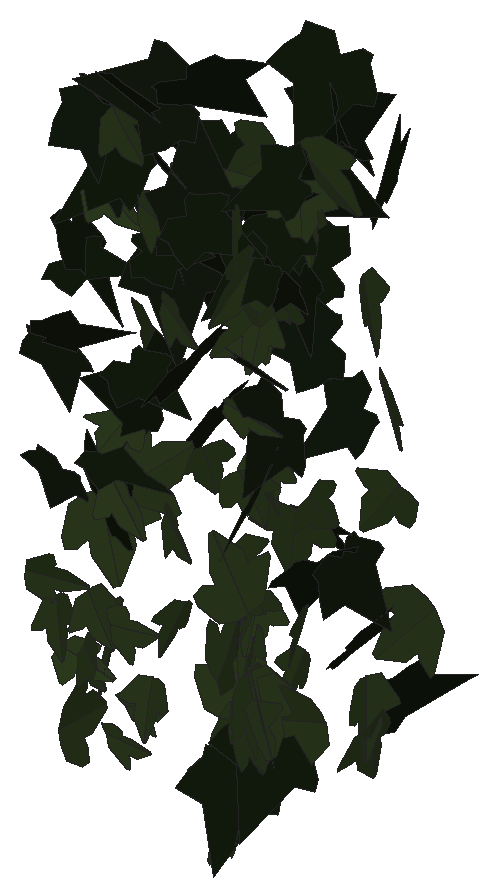
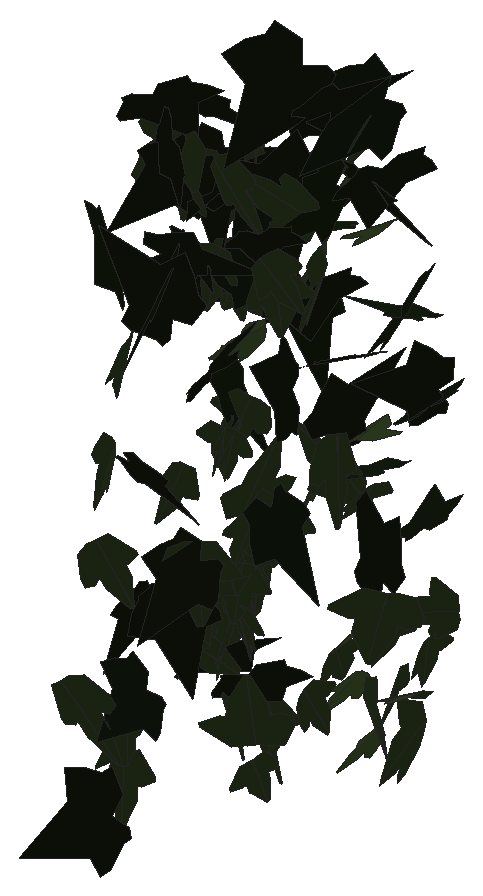
# SketchUp Ruby script. Lengths in inches.
U = 1.inch
M = Sketchup.active_model
def pt(a) = Geom::Point3d.new(a.map { |v| v * U })
def face(e, loops, mat)
  f = e.add_face(loops[0].map { |a| pt(a) })
  loops[1..].each { |l| e.add_face(l.map { |a| pt(a) }).erase! }
  f.material = f.back_material = mat if mat
  f
end
# faces: each face lists its corners as indices into pts; further lists are holes
def faces(e, pts, list, mat = nil) = list.each { |f| face(e, (f[0].is_a?(Array) ? f : [f]).map { |l| l.map { |i| pts[i] } }, mat) }
# xy, xz, yz: faces in a plane at the given z, y or x. An outline is a flat list of corners, or four numbers for a rectangle; further outlines are holes
def ring(l) = l.size == 4 ? [[l[0], l[1]], [l[2], l[1]], [l[2], l[3]], [l[0], l[3]]] : l.each_slice(2).to_a
def flat(e, list, mat, &to3) = list.each { |f| face(e, (f[0].is_a?(Array) ? f : [f]).map { |l| ring(l).map { |u, v| to3.(u, v) } }, mat) }
def xy(e, z, list, mat = nil) = flat(e, list, mat) { |x, y| [x, y, z] }
def xz(e, y, list, mat = nil) = flat(e, list, mat) { |x, z| [x, y, z] }
def yz(e, x, list, mat = nil) = flat(e, list, mat) { |y, z| [x, y, z] }
def lines(e, pts, list) = list.each { |a, b| e.add_line(pt(pts[a]), pt(pts[b])) }
# prism: a flat outline (further loops are holes) pulled along v
def prism(e, loops, v, mat = nil)
  f = face(e, loops, mat); d = Geom::Vector3d.new(v.map { |x| x * U })
  f.pushpull(f.normal.samedirection?(d) ? d.length : -d.length)
end
def box(e, o, s, mat = nil) = prism(e, [[o, [o[0] + s[0], o[1], o[2]], [o[0] + s[0], o[1] + s[1], o[2]], [o[0], o[1] + s[1], o[2]]]], [0, 0, s[2]], mat)
def at(x, y, z, deg = 0) = Geom::Transformation.translation(pt([x, y, z])) * Geom::Transformation.rotation(ORIGIN, Z_AXIS, deg.degrees)
def axes(o, x, y, z) = Geom::Transformation.new([*x, 0, *y, 0, *z, 0, *pt(o).to_a, 1])
def part(name) = M.definitions.add(name)
# library, detail: a bought-in or finely detailed component or shape, given as its bounding box
def library(name, o, s) = part(name).tap { |d| box(d.entities, o, s) }
def detail(e, o, s) = box(e.add_group.entities, o, s)
def put(e, d, t, mat = nil) = e.add_instance(d, t).tap { |i| i.material = mat if mat }
def group(e, t, mat = nil) = e.add_group.tap { |g| g.transformation = t; g.material = mat if mat }.entities
root = M.entities
M.materials.add("efeu1").color = [18, 25, 13]
M.materials.add("efeu2").color = [43, 57, 29]
c1 = part("ivyleaf_10")
p = [[0,0.5,-0.03],[-0.0625,2.02,-0.43],[-0.19,2.01,-0.46],[-0.54,1.05,-0.29],[-0.52,0.625,-0.18],[-0.83,0.76,-0.28],
  [-1.16,0.64,-0.33],[-1.15,0.33,-0.24],[-0.77,-0.39,0.02],[-0.3,-0.51,0.16],[0.04,-0.48,0.23],[-0.02,2.01,-0.4375],
  [-0.06,2.01,-0.43],[0.04,-0.49,0.23],[0.67,-0.49,0.14],[1.38,0.36,-0.2],[1.375,0.51,-0.24],[0.81,0.65,-0.19],
  [0.62,0.59,-0.15],[0.6,1.09,-0.28],[0.5,1.23,-0.31]]
faces(c1.entities,p,[[0,1,2,3,4,5,6,7,8,9,10],[11,12,0,13,14,15,16,17,18,19,20]],"efeu2")
c2 = part("ivyleaf_9")
p = [[1.54,2.16,1.25],[1.36,2.04,1.19],[-0.21,0.99,0.68],[-0.71,1.11,0.82],[-0.85,0.86,0.67],[-0.8,0.17,0.21],
  [-0.9,-0.01,0.1],[-0.67,-0.16,-0.02],[-0.08,-0.08,-0.05],[-0.03,-0.6,-0.4],[0.65,-0.88,-0.66],[0.83,-0.6,-0.49],
  [1.29,-0.42,-0.43],[1.8125,-0.07,-0.26],[1.21,0.44,0.15]]
faces(c2.entities,p,[[0,1,2,3,4,5,6,7,8,9,10,11,12,13,14]],"efeu1")
put(root,c1,axes([586.05,128.29,189.875],[0.13777,-0.1156,0.68429],[0.55453,0.4378,-0.03769],[-0.41727,0.54365,0.17585]))
put(root,c1,axes([586.36,128.71,188.74],[-0.02608,-0.71977,0.14562],[0.34937,-0.14032,-0.63103],[0.64591,0.04684,0.3472]))
put(root,c2,axes([586.13,129.02,196.92],[0.02994,-0.77843,0.19838],[0.30223,-0.17302,-0.72452],[0.74429,0.10157,0.28622]))
put(root,c2,axes([586.26,129.04,192.97],[-0.21332,-0.59102,0.45433],[0.308,-0.50022,-0.5061],[0.67886,0.04124,0.37238]))
put(root,c2,axes([586.15,128.7,197.34],[0.47444,0.02155,0.66199],[0.63643,0.21069,-0.46298],[-0.18344,0.78673,0.10585]))
put(root,c1,axes([586.41,130.7,191.02],[0.78115,0.73417,0.24902],[0.18487,0.16692,-1.072],[-0.75289,0.80271,-0.00485]))
put(root,c1,axes([587.17,132.04,196.33],[-0.85539,0.2797,0.52223],[-0.49092,0.17874,-0.89983],[-0.3316,-0.98614,-0.01498]))
put(root,c2,axes([586.34,129.57,200.51],[0.65227,-0.79795,-0.17464],[-0.10982,0.1358,-1.03062],[0.80942,0.66145,0.00091]))
put(root,c1,axes([586.71,130.87,187.58],[0.69898,-0.74224,0.39536],[0.26843,-0.29029,-1.01955],[0.79698,0.74875,-0.00336]))
put(root,c1,axes([587.25,128.31,185.47],[-0.07423,0.16774,1.11083],[-0.49986,0.99205,-0.1832],[-1.00609,-0.50526,0.00907]))
put(root,c1,axes([586.64,129.05,187.25],[0.01692,-0.64732,-0.23753],[0.67208,0.06858,-0.13903],[0.1541,-0.22804,0.63244]))
put(root,c2,axes([586.54,129.05,199.8],[0.55427,-0.51643,-0.1309],[0.45505,0.55715,-0.27124],[0.27707,0.11807,0.70735]))
put(root,c1,axes([587.25,128.96,187.52],[0.25073,-0.64179,-0.17543],[0.26152,0.26745,-0.60466],[0.61178,0.1487,0.33037]))
put(root,c2,axes([586.82,130.28,191.63],[-0.13016,-0.00362,1.19027],[0.56176,-1.05581,0.05822],[1.04937,0.56476,0.11648]))
put(root,c2,axes([587.21,129.76,204.62],[-0.10832,-1.02535,-0.37043],[0.03645,0.36864,-1.03105],[1.0896,-0.11427,-0.00234]))
put(root,c1,axes([587.44,128.96,189.1875],[-0.05976,-0.73491,-0.09625],[0.43185,0.04395,-0.60374],[0.60238,-0.10442,0.42327]))
put(root,c1,axes([588.15,131.93,187.85],[-0.00093,-0.60937,0.30873],[0.04157,-0.30821,-0.60822],[0.68185,0.01797,0.0375]))
put(root,c2,axes([588.63,129.31,203.83],[-1.09293,0.11233,-0.02551],[0.01922,-0.06221,-1.09706],[-0.11357,-1.09146,0.0599]))
put(root,c1,axes([588.66,133.1,202.34],[0.48228,0.09622,-0.59732],[-0.59134,0.23653,-0.43934],[0.12797,0.73037,0.22098]))
put(root,c1,axes([587.73,129.0625,202.3],[0.02053,-0.78461,-0.03553],[0.75258,0.02982,-0.22368],[0.22472,-0.02819,0.75233]))
put(root,c1,axes([588.43,129.09,195.15],[-0.6903,-0.14918,0.224],[0.19282,-0.70434,0.12516],[0.18774,0.17491,0.69505]))
put(root,c2,axes([588.86,132.73,194.125],[-0.47604,0.80347,-0.50065],[0.23512,-0.44248,-0.93368],[-0.91702,-0.53054,0.0205]))
put(root,c1,axes([588.3,128.86,185.18],[0.52006,-0.39557,-0.21933],[0.30808,0.5545,-0.26956],[0.33116,0.10536,0.59521]))
put(root,c2,axes([587.97,128.91,194.15],[0.46394,-0.60081,-0.1519],[0.37966,0.42553,-0.52352],[0.48981,0.23925,0.54968]))
put(root,c2,axes([588.8125,130.11,195.7],[-0.01816,-0.01498,1.10733],[-0.71725,-0.84365,-0.02318],[0.84377,-0.71747,0.00413]))
put(root,c1,axes([588.78,132.73,201.58],[-0.57493,-0.49623,0.11289],[-0.03338,-0.13318,-0.75543],[0.50781,-0.57057,0.07815]))
put(root,c2,axes([587.9,133.13,198.65],[0.28392,-0.11605,-1.00857],[1.01522,0.03577,0.28167],[0.00321,-1.04716,0.12139]))
put(root,c2,axes([588.2,128.67,206.07],[1.12084,0.05707,0.01287],[0.01107,0.03564,-1.12175],[-0.05745,1.12035,0.03503]))
put(root,c1,axes([588.54,128.7,205.13],[0.09649,-0.7933,-0.18292],[0.45075,0.20545,-0.65323],[0.67795,-0.02369,0.46035]))
put(root,c1,axes([588.58,128.72,188.88],[0.46426,-0.3966,-0.40602],[0.32133,0.61605,-0.23433],[0.46785,-0.02956,0.56385]))
put(root,c1,axes([588.48,128.8,193.16],[-0.14155,-0.72801,-0.0542],[0.57266,-0.07649,-0.46817],[0.45276,-0.13085,0.5752]))
put(root,c1,axes([588.9,130.625,200.91],[-0.6167,0.84837,-0.22552],[0.15082,-0.16911,-1.0486],[-0.86478,-0.63449,-0.02206]))
put(root,c2,axes([589.65,130.02,205.68],[-0.12174,-0.90105,-0.60518],[-0.09557,-0.59771,0.90915],[-1.0812,0.15429,-0.01222]))
put(root,c1,axes([589.28,131.74,193.35],[-0.38397,-0.59309,-0.15346],[0.11431,0.10857,-0.70561],[0.60186,-0.399,0.03611]))
put(root,c1,axes([589.1875,128.57,186.6],[0.5933,-0.23635,-0.26569],[0.18712,0.64698,-0.1577],[0.30239,0.06339,0.61887]))
put(root,c2,axes([588.93,129.92,203.5625],[1.04486,-0.33971,-0.04287],[-0.04218,0.00891,-1.09869],[0.3398,1.04571,-0.00457]))
put(root,c2,axes([589.33,132.72,203.03],[-0.33806,-0.65558,-0.25431],[0.18801,0.18763,-0.73361],[0.67757,-0.37915,0.07668]))
put(root,c2,axes([589.27,130.45,200.19],[-0.17654,-1.02923,-0.21362],[0.03699,0.21039,-1.04426],[1.05052,-0.18037,0.00088]))
put(root,c2,axes([589.08,128.72,197.41],[0.32391,-0.6182,-0.31947],[0.34025,0.44809,-0.5221],[0.60701,0.07871,0.46313]))
put(root,c1,axes([588.9375,129.29,193.625],[0.67907,-0.13297,-0.79694],[0.79162,-0.09878,0.69102],[-0.16165,-1.04235,0.03618]))
put(root,c1,axes([589.71,128.68,187.3],[-0.20403,-0.588,0.33927],[0.32561,-0.39561,-0.48984],[0.59568,0.01485,0.38396]))
put(root,c1,axes([589.67,128.5625,202.63],[0.43747,-0.56137,-0.35728],[0.3332,0.55491,-0.46391],[0.57599,0.10536,0.53972]))
put(root,c2,axes([589.8,136.45,203.11],[0.75781,-0.50642,-0.66784],[-0.55853,0.36617,-0.91143],[0.62491,0.94139,-0.00475]))
put(root,c2,axes([589.73,128.52,201.375],[0.73576,-0.18714,-0.20691],[0.0998,0.72152,-0.2977],[0.26053,0.25211,0.69839]))
put(root,c2,axes([589.65,136.52,202.01],[-0.06323,-0.05609,1.12568],[0.9616,-0.59077,0.02457],[0.58789,0.96028,0.08087]))
put(root,c1,axes([590.36,131.73,185.89],[0.93344,0.55515,-0.12163],[0.08905,0.08812,1.08564],[0.5613,-0.9372,0.03003]))
put(root,c1,axes([589.8125,130.32,202.53],[0.3925,-0.06622,-1.01584],[1.01558,-0.04945,0.39562],[-0.07005,-1.0879,0.04385]))
put(root,c1,axes([590.48,128.57,192.98],[0.36868,-0.63247,-0.12508],[0.3146,0.30226,-0.60105],[0.56275,0.24539,0.41795]))
put(root,c2,axes([591.0625,129.26,202.32],[-1.14149,-0.10172,0.28438],[0.29042,-0.06455,1.14267],[-0.08289,1.17461,0.08742]))
put(root,c2,axes([590.49,129.54,206.7],[0.81903,0.87426,0.24465],[0.16851,0.17738,-1.19797],[-0.89207,0.83619,-0.00167]))
put(root,c1,axes([590.73,128.23,199.96],[0.4211,-0.63505,-0.13307],[0.38926,0.37418,-0.55389],[0.51911,0.23457,0.52328]))
put(root,c1,axes([591.51,131.55,203.77],[0.65074,-0.37421,-0.7487],[-0.66145,0.35123,-0.75045],[0.5129,0.92772,-0.01788]))
put(root,c2,axes([591.49,128.12,198.69],[-0.28552,1.10913,-0.1052],[0.02765,-0.10151,-1.14529],[-1.11377,-0.28685,-0.00146]))
put(root,c1,axes([591.19,130.65,183.99],[0.20398,0.59083,-0.20369],[-0.17534,-0.15155,-0.6152],[-0.59985,0.24521,0.11056]))
put(root,c1,axes([591.17,130.22,185.76],[0.54309,-0.39053,0.07419],[0.07251,-0.02619,-0.6686],[0.39085,0.54751,0.02094]))
put(root,c1,axes([591.41,129.73,185.25],[-0.37006,-0.55743,-0.02026],[0.01047,0.01737,-0.66908],[0.5577,-0.3702,-0.00088]))
put(root,c1,axes([591.66,132.8,191.61],[-0.89097,-0.38537,0.17041],[-0.132,-0.12326,-0.96889],[0.40016,-0.8987,0.05981]))
put(root,c1,axes([591.39,130.53,186.2],[0.62113,-0.25645,0.01845],[0.02071,0.00182,-0.67192],[0.25627,0.6214,0.00959]))
put(root,c1,axes([591.71,130.02,190.71],[-0.50006,0.4695,0.16327],[-0.16888,0.05736,-0.68216],[-0.46752,-0.5229,0.07177]))
put(root,c2,axes([591.41,133.0625,191.66],[0.9194,0.31654,-0.15049],[-0.1971,0.11759,-0.9568],[-0.28983,0.92418,0.17328]))
put(root,c1,axes([591.73,130.6875,190.12],[-0.63101,-0.29889,-0.0219],[0.01804,0.01306,-0.69821],[0.29915,-0.63126,-0.00408]))
put(root,c2,axes([590.97,130.36,200.35],[1.19253,-0.08387,-0.27225],[0.27139,-0.02173,1.19547],[-0.0866,-1.22302,-0.00257]))
put(root,c1,axes([591.83,130.93,185.69],[0.44027,-0.40444,-0.31148],[-0.20446,0.23719,-0.59697],[0.46775,0.48436,0.03224]))
put(root,c1,axes([591.64,130.63,188.6],[0.5263,-0.41905,0.14553],[0.12742,-0.07348,-0.67241],[0.42491,0.54108,0.02139]))
put(root,c1,axes([591.6875,130.67,188.92],[0.6654,-0.18185,0.0303],[0.0285,-0.01064,-0.6898],[0.18214,0.66601,-0.00275]))
put(root,c1,axes([591.74,130.23,191.66],[0.00038,0.65668,0.27499],[-0.06837,0.27376,-0.65363],[-0.70864,-0.02606,0.06321]))
put(root,c1,axes([591.8,130.83,189.76],[0.48171,0.48315,-0.13559],[-0.10284,-0.08891,-0.68219],[-0.49117,0.49247,0.00986]))
put(root,c2,axes([592.14,133.125,190.22],[0.12005,0.89185,-0.37066],[-0.11817,-0.35714,-0.8976],[-0.95855,0.15573,0.06423]))
put(root,c1,axes([592.24,129.09,191.43],[0.21223,-0.04077,-0.67789],[-0.4693,0.50456,-0.17727],[0.49088,0.5,0.12361]))
put(root,c1,axes([591.79,130.29,190.45],[0.6759,-0.17246,0.09423],[0.09296,-0.0168,-0.69752],[0.17315,0.68223,0.00664]))
put(root,c2,axes([591.35,128.43,203.07],[0.39277,-0.43328,-0.55246],[0.33174,0.67244,-0.29152],[0.61878,-0.08549,0.50696]))
put(root,c1,axes([591.97,129.75,189.73],[0.41568,-0.50478,-0.24792],[-0.0352,0.28433,-0.63794],[0.56127,0.39167,0.1436]))
put(root,c1,axes([591.55,129.53,185.12],[0.43241,-0.50984,-0.0235],[0.51036,0.43219,0.01431],[0.00428,-0.02717,0.66836]))
put(root,c1,axes([592.31,130.02,199.22],[0.51249,0.16623,-0.53106],[-0.5226,-0.10427,-0.53696],[-0.19118,0.73062,0.0442]))
put(root,c1,axes([591.81,130.79,185.48],[0.51009,-0.18841,0.39341],[0.38223,-0.09858,-0.54281],[0.21016,0.63659,0.03238]))
put(root,c1,axes([592.22,130.33,194.28],[-0.26185,0.67831,-0.02394],[0.00388,-0.02416,-0.72708],[-0.67872,-0.26183,0.00508]))
put(root,c1,axes([592.47,128.34,189.19],[0.01751,0.40215,-0.91438],[-0.09019,0.91142,0.39912],[0.99483,0.07555,0.05228]))
put(root,c2,axes([592.8,134.2,194.92],[-0.88282,0.07844,0.0797],[-0.07909,0.01043,-0.88629],[-0.07906,-0.88635,-0.00338]))
put(root,c1,axes([592.22,130.73,194.57],[0.71445,0.10714,0.07421],[0.06171,0.0861,-0.71847],[-0.1148,0.71312,0.0756]))
put(root,c1,axes([592.52,128.78,184.51],[0.80501,-0.64729,-0.2514],[-0.19611,0.1573,-1.03297],[0.66613,0.82856,-0.00029]))
put(root,c1,axes([592.5,129.94,200.125],[-0.73922,-0.1771,-0.04806],[0.04397,0.02274,-0.76005],[0.17816,-0.74044,-0.01185]))
put(root,c1,axes([592.44,130.39,194.54],[-0.32032,0.64019,0.12914],[-0.04323,0.12274,-0.71568],[-0.65165,-0.32283,-0.016]))
put(root,c2,axes([592.1875,136.14,184.4375],[0.42315,0.56634,0.87028],[0.5277,0.69207,-0.70694],[-0.89424,0.67638,-0.00536]))
put(root,c1,axes([592.47,130.07,199.4],[0.7576,0.01182,-0.00148],[-0.00148,0.00001,-0.75769],[-0.01182,0.7576,0.00003]))
put(root,c2,axes([592.65,133.92,187.4],[0.30197,0.62954,0.63039],[0.1013,0.63704,-0.6847],[-0.88513,0.28768,0.13671]))
put(root,c2,axes([593.4,131.97,200.66],[-0.7356,0.05233,0.71313],[-0.71484,-0.078,-0.73164],[0.0169,-1.02155,0.0924]))
put(root,c1,axes([592.78,130.49,200.06],[-0.75668,0.09692,0.02534],[-0.02567,-0.00091,-0.76285],[-0.09684,-0.7571,0.00416]))
put(root,c1,axes([592.82,128.76,191.35],[0.17805,1.02887,0.22739],[-0.04868,-0.22234,1.04411],[1.05257,-0.18432,0.00983]))
put(root,c1,axes([592.6,128.9,203.25],[-0.4011,0.46963,-0.48216],[0.14694,-0.48664,-0.59624],[-0.65684,-0.39565,0.16104]))
put(root,c2,axes([592.82,133.18,206.6],[-0.63802,-0.87666,-0.02225],[0.01293,0.01811,-1.08425],[0.87685,-0.63815,-0.0002]))
put(root,c1,axes([592.61,129.21,194.7],[0.61118,0.27456,0.29436],[0.13563,0.36341,-0.62057],[-0.379,0.57282,0.25261]))
put(root,c2,axes([592.29,133.1,205.3],[-0.25736,0.01277,-1.04929],[1.04922,-0.01471,-0.25752],[-0.01733,-1.08029,-0.0089]))
put(root,c2,axes([592.8,128.83,185.61],[-0.5242,-0.82587,-0.14831],[0.08321,0.12284,-0.97817],[0.83494,-0.53074,0.00438]))
put(root,c1,axes([593.36,134.98,192.12],[-0.66438,-0.15305,0.53219],[-0.4783,-0.26031,-0.67196],[0.27908,-0.81048,0.11532]))
put(root,c2,axes([592.875,130.05,203.41],[0.45203,0.63355,0.07066],[0.01349,0.0771,-0.77755],[-0.63733,0.45097,0.03367]))
put(root,c1,axes([592.83,129.68,187.91],[-0.5605,0.95467,-0.11474],[0.05162,-0.10275,-1.10702],[-0.96015,-0.56283,0.00746]))
put(root,c2,axes([592.8,133.51,190.39],[0.22043,-0.55459,-0.74191],[-0.2925,0.68193,-0.59666],[0.87889,0.36604,-0.0125]))
put(root,c1,axes([592.51,129,197.05],[0.43364,-0.60691,0.00737],[0.57482,0.40774,-0.24448],[0.19489,0.1478,0.70471]))
put(root,c2,axes([593.41,134.54,201.84],[0.00925,0.42481,1.04329],[-0.12993,1.03676,-0.421],[-1.11894,-0.11687,0.05751]))
put(root,c2,axes([593.36,129.07,201.97],[-0.73244,-0.23662,0.09114],[-0.09234,-0.01055,-0.7695],[0.23615,-0.73802,-0.01822]))
put(root,c1,axes([592.95,131.28,188.21],[-0.02807,-0.4918,0.49669],[0.23826,-0.47405,-0.45592],[0.65711,0.15088,0.18653]))
put(root,c1,axes([593.02,134.29,198.76],[-0.31033,0.85759,-0.09989],[0.01234,-0.10173,-0.91172],[-0.8633,-0.30973,0.02288]))
put(root,c1,axes([593.04,131.3125,189.63],[0.31811,-0.57434,0.26629],[0.13706,-0.22847,-0.6565],[0.61806,0.34628,0.00853]))
put(root,c1,axes([593.17,128.85,201.84],[0.06329,0.53285,-0.84283],[-0.22699,-0.81465,-0.53209],[-0.97096,0.22518,0.06945]))
put(root,c2,axes([593.05,130.54,202.51],[-0.39666,-0.65537,-0.12926],[0.07999,0.10266,-0.76591],[0.66319,-0.40436,0.01506]))
put(root,c1,axes([593.21,134.08,184.76],[-0.04184,-0.86716,-0.26414],[0.04024,0.26238,-0.86776],[0.9056,-0.05172,0.02635]))
put(root,c1,axes([593.59,135.88,187.8],[0.85766,-0.24016,-0.69333],[-0.66466,0.19749,-0.89061],[0.31081,1.08503,0.00864]))
put(root,c1,axes([593.05,129.14,188.16],[-0.00158,1.1336,-0.02411],[0.00478,-0.0241,-1.13359],[-1.13385,-0.00169,-0.00474]))
put(root,c1,axes([593.12,134.17,185.98],[-0.00514,0.90595,-0.20035],[-0.05004,-0.20033,-0.90459],[-0.92649,0.00579,0.04997]))
put(root,c2,axes([593,130.43,196.33],[-0.15359,-0.87286,0.61171],[-0.08008,-0.60683,-0.886],[1.06285,-0.17185,0.02164]))
put(root,c1,axes([593.23,134.87,195.375],[-0.65498,0.59718,-0.04404],[0.01626,-0.0475,-0.88602],[-0.59858,-0.65473,0.02412]))
put(root,c1,axes([593.18,131.62,193.28],[-0.11534,-0.57536,-0.43118],[0.20203,0.39317,-0.57867],[0.69003,-0.21129,0.09735]))
put(root,c1,axes([593.1,129.25,187.92],[0.21034,1.10925,0.00632],[0.00319,0.00583,-1.12901],[-1.10926,0.21036,-0.00205]))
put(root,c2,axes([593.51,129.13,195.43],[-0.72117,0.54407,-0.54667],[0.43958,-0.32502,-0.90338],[-0.63375,-0.84457,-0.00451]))
put(root,c2,axes([593.05,131.45,203.6],[0.02032,-0.08776,-1.04254],[-0.06117,1.04085,-0.08881],[1.04444,0.06266,0.01508]))
put(root,c1,axes([593.29,128.63,187.41],[-0.04274,0.8381,0.37468],[-0.0468,0.37261,-0.83881],[-0.91685,-0.05809,0.02535]))
put(root,c1,axes([594.1,130.25,187.14],[0.28853,0.0285,-0.97971],[-0.95641,0.23149,-0.27493],[0.21431,0.99473,0.09206]))
put(root,c2,axes([593.66,129.42,201.67],[0.46657,0.19365,-0.59397],[-0.5681,-0.17694,-0.50393],[-0.25994,0.73429,0.03521]))
put(root,c2,axes([593.95,129.83,204.63],[-0.74159,-0.01628,0.27354],[-0.27184,-0.05581,-0.74029],[0.03456,-0.78845,0.04676]))
put(root,c2,axes([593.46,129.23,198.42],[-0.59872,-0.19802,0.43041],[0.22702,-0.72871,-0.01945],[0.41584,0.11273,0.63032]))
put(root,c1,axes([593.29,130.84,203.43],[0.65235,0.41606,0.08613],[0.0625,0.06212,-0.77351],[-0.42026,0.65508,0.01865]))
put(root,c2,axes([593.11,131.125,200.53],[-0.30658,-0.18502,-0.67314],[0.67835,0.0947,-0.33498],[0.1649,-0.73358,0.12654]))
put(root,c1,axes([593.1875,131.31,202.72],[0.6822,-0.17258,0.32283],[0.32001,-0.05037,-0.70318],[0.17775,0.75305,0.02695]))
put(root,c2,axes([594.2,130.91,199.1],[-0.34641,-0.35025,-0.80445],[-0.53929,-0.59722,0.49225],[-0.69208,0.64068,0.01908]))
put(root,c2,axes([593.41,129.78,186.46],[-0.49215,-0.97903,0.15984],[0.10766,-0.23009,-1.07783],[0.98613,-0.46349,0.19745]))
put(root,c1,axes([593.17,131.59,204.3],[-0.79782,0.07041,-0.65551],[0.65259,-0.06194,-0.80091],[-0.09372,-1.03071,0.00335]))
